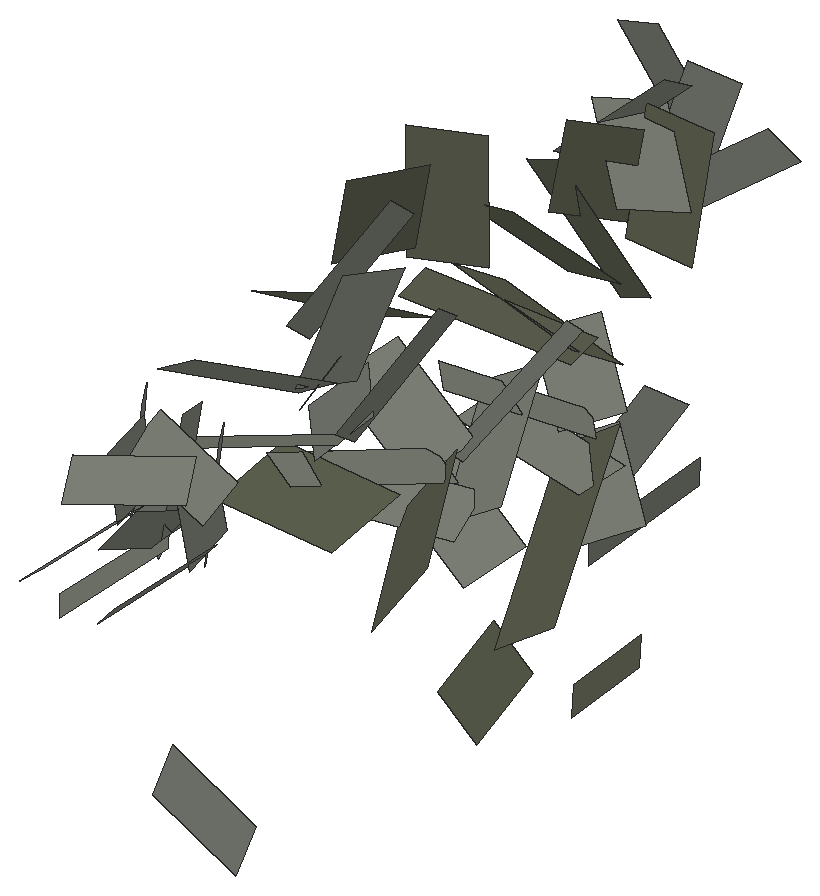
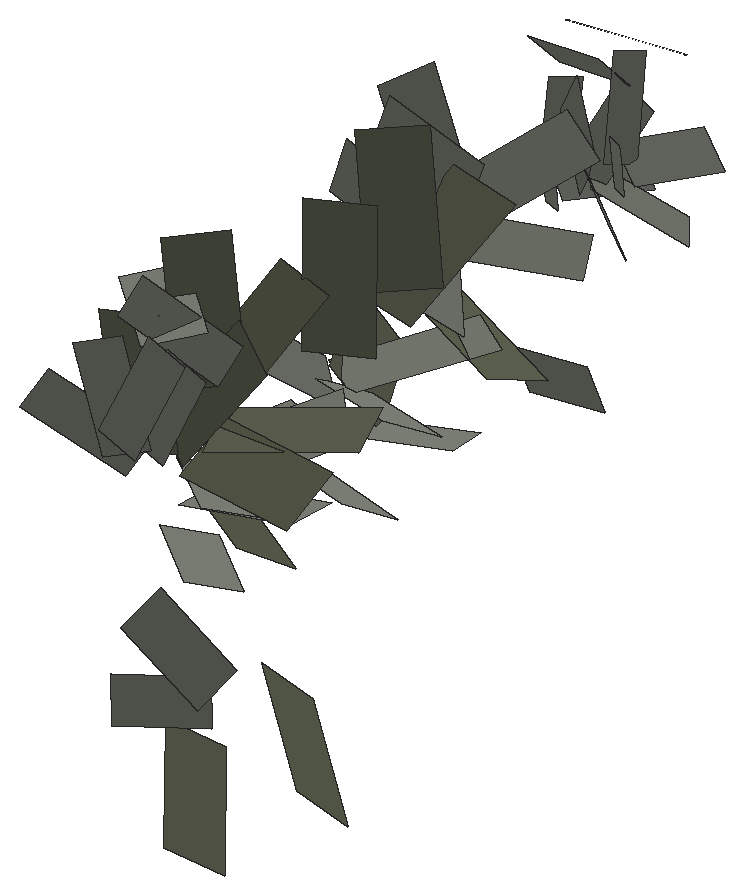
# SketchUp Ruby script. Lengths in inches.
U = 1.inch
M = Sketchup.active_model
def pt(a) = Geom::Point3d.new(a.map { |v| v * U })
def face(e, loops, mat)
  f = e.add_face(loops[0].map { |a| pt(a) })
  loops[1..].each { |l| e.add_face(l.map { |a| pt(a) }).erase! }
  f.material = f.back_material = mat if mat
  f
end
# faces: each face lists its corners as indices into pts; further lists are holes
def faces(e, pts, list, mat = nil) = list.each { |f| face(e, (f[0].is_a?(Array) ? f : [f]).map { |l| l.map { |i| pts[i] } }, mat) }
# xy, xz, yz: faces in a plane at the given z, y or x. An outline is a flat list of corners, or four numbers for a rectangle; further outlines are holes
def ring(l) = l.size == 4 ? [[l[0], l[1]], [l[2], l[1]], [l[2], l[3]], [l[0], l[3]]] : l.each_slice(2).to_a
def flat(e, list, mat, &to3) = list.each { |f| face(e, (f[0].is_a?(Array) ? f : [f]).map { |l| ring(l).map { |u, v| to3.(u, v) } }, mat) }
def xy(e, z, list, mat = nil) = flat(e, list, mat) { |x, y| [x, y, z] }
def xz(e, y, list, mat = nil) = flat(e, list, mat) { |x, z| [x, y, z] }
def yz(e, x, list, mat = nil) = flat(e, list, mat) { |y, z| [x, y, z] }
def lines(e, pts, list) = list.each { |a, b| e.add_line(pt(pts[a]), pt(pts[b])) }
# prism: a flat outline (further loops are holes) pulled along v
def prism(e, loops, v, mat = nil)
  f = face(e, loops, mat); d = Geom::Vector3d.new(v.map { |x| x * U })
  f.pushpull(f.normal.samedirection?(d) ? d.length : -d.length)
end
def box(e, o, s, mat = nil) = prism(e, [[o, [o[0] + s[0], o[1], o[2]], [o[0] + s[0], o[1] + s[1], o[2]], [o[0], o[1] + s[1], o[2]]]], [0, 0, s[2]], mat)
def at(x, y, z, deg = 0) = Geom::Transformation.translation(pt([x, y, z])) * Geom::Transformation.rotation(ORIGIN, Z_AXIS, deg.degrees)
def axes(o, x, y, z) = Geom::Transformation.new([*x, 0, *y, 0, *z, 0, *pt(o).to_a, 1])
def part(name) = M.definitions.add(name)
# library, detail: a bought-in or finely detailed component or shape, given as its bounding box
def library(name, o, s) = part(name).tap { |d| box(d.entities, o, s) }
def detail(e, o, s) = box(e.add_group.entities, o, s)
def put(e, d, t, mat = nil) = e.add_instance(d, t).tap { |i| i.material = mat if mat }
def group(e, t, mat = nil) = e.add_group.tap { |g| g.transformation = t; g.material = mat if mat }.entities
root = M.entities
M.materials.add("viburnumblaasdfas0df1w06d").color = [98, 102, 84]
M.materials.add("viburnumbladsadfasdfad0w122").color = [125, 129, 119]
c1 = part("Component\#314")
p = [[0.14,0,0],[2.58,0.05,0.25],[2.44,5.11,2.64],[0,5.05,2.39]]
faces(c1.entities,p,[[0,1,2,3]],"viburnumblaasdfas0df1w06d")
c2 = part("viburnumblad1\#2")
put(c2.entities,c1,axes([-37.25,6.23,19.31],[75.98784,0,0],[0,65.50676,0],[0,0,75.98784]))
c3 = part("Component\#315")
p = [[0.25,0,0],[2.05,0.01,0.35],[1.81,4.2,1.66],[0,4.19,1.3125]]
faces(c3.entities,p,[[0,1,2,3]],"viburnumbladsadfasdfad0w122")
c4 = part("viburnumblad2")
put(c4.entities,c3,axes([-19.23,-4.49,-32.18],[83.35428,0,0],[0,79.38502,0],[0,0,83.35428]))
put(root,c2,axes([2194.68,269.67,26.76],[-0.01129,-0.00613,-0.00067],[0.00417,-0.00777,0.01127],[-0.0047,0.00912,0.00614]))
put(root,c4,axes([2194.36,254.17,25.81],[0.0062,-0.00344,0.00762],[-0.00192,0.00879,0.00527],[-0.00787,-0.00449,0.00364]))
put(root,c4,axes([2195.61,279.33,28.08],[-0.00984,-0.00064,-0.00419],[-0.00322,-0.006,0.00808],[-0.00275,0.0086,0.00434]))
put(root,c2,axes([2197.04,271.39,24.12],[0.00188,0.00994,-0.00772],[-0.0143,-0.00023,-0.00375],[-0.00243,0.00751,0.00854]))
put(root,c2,axes([2193.96,267.38,28.05],[-0.00729,-0.01049,-0.00199],[0.00959,-0.00792,0.00787],[-0.00649,0.00328,0.00895]))
put(root,c2,axes([2197.38,270.9375,24.14],[-0.00372,0.0118,-0.00306],[-0.01362,-0.00502,-0.00283],[-0.00309,0.00191,0.01102]))
put(root,c2,axes([2196.67,267.9,13.27],[0.00499,0.00892,0.00903],[-0.00667,0.01209,-0.00778],[-0.01141,-0.0013,0.00685]))
put(root,c2,axes([2195.66,266.375,26.96],[-0.01203,-0.00093,-0.00471],[0.00029,-0.01476,0.00205],[-0.00435,0.00215,0.01023]))
put(root,c4,axes([2196.07,264.76,23.18],[0.00718,0.01175,0.00394],[-0.01195,0.00776,-0.0014],[-0.003,-0.00258,0.01303]))
put(root,c4,axes([2195.62,253.83,25.125],[0.00371,0.00412,0.00878],[-0.006,0.0085,-0.00147],[-0.00737,-0.00446,0.00446]))
put(root,c4,axes([2195.48,253.28,27.01],[-0.0062,0.00344,-0.00762],[-0.00004,-0.00961,-0.00424],[-0.0081,-0.00223,0.0048]))
put(root,c4,axes([2196.2,277.29,26.83],[-0.01027,-0.00067,-0.00437],[-0.0029,-0.0054,0.00727],[-0.00275,0.0086,0.00434]))
put(root,c4,axes([2197.32,259.9,26.98],[-0.00427,0.01006,-0.00619],[-0.01054,-0.00775,-0.00533],[-0.00749,0.00313,0.01026]))
put(root,c4,axes([2196.43,253.22,26],[-0.00506,0.00898,-0.002],[-0.00471,-0.00455,-0.00828],[-0.00753,-0.00286,0.00529]))
put(root,c4,axes([2196.67,260.61,28.44],[-0.00935,0.0021,-0.00891],[-0.00409,-0.01235,0.00138],[-0.00819,0.00377,0.00948]))
put(root,c4,axes([2197.66,264.6875,21.89],[-0.00305,0.01398,0.00068],[-0.01364,-0.00282,-0.0033],[-0.00279,-0.00128,0.01326]))
put(root,c4,axes([2194.46,275.59,16.81],[-0.00173,-0.0098,0.00563],[0.00735,0.00343,0.00822],[-0.00865,0.00481,0.00572]))
put(root,c4,axes([2194.93,254.49,26.95],[0.00095,-0.00927,-0.00479],[0.00517,-0.00382,0.00808],[-0.00874,-0.00294,0.00329]))
put(root,c4,axes([2194.1,275.0625,28.37],[0.00162,-0.00936,0.00394],[0.00963,0.00389,0.00496],[-0.00566,0.00263,0.0077]))
put(root,c2,axes([2197.62,273.6,25.08],[-0.00938,0.00386,-0.00599],[-0.00819,-0.00718,0.008],[-0.00057,0.00892,0.00623]))
put(root,c2,axes([2198.51,259.2,23.77],[0.00387,0.01311,0.00437],[-0.0121,0.00667,-0.00928],[-0.00906,-0.00102,0.01108]))
put(root,c4,axes([2197.77,264.79,23.78],[-0.01149,0.00801,-0.00297],[-0.00766,-0.01186,-0.00235],[-0.00352,-0.00017,0.01315]))
put(root,c4,axes([2196.13,260.3125,25.88],[0.00916,0.00784,0.00642],[-0.00492,0.00961,-0.00471],[-0.00802,0.00094,0.01029]))
put(root,c4,axes([2195.07,261.02,26.84],[0.00935,-0.0021,0.00891],[0.00182,0.01184,0.00088],[-0.00893,0.00067,0.00953]))
put(root,c4,axes([2194.54,262.14,28.43],[0.00445,-0.01048,0.00645],[0.00766,0.00772,0.00727],[-0.00963,0.0013,0.00876]))
put(root,c4,axes([2194.7,274.57,15.69],[0.00508,-0.00494,0.00777],[0.00608,0.00946,0.00204],[-0.00795,0.00351,0.00743]))
put(root,c2,axes([2197.29,272.64,25.9],[-0.0112,0.0013,-0.00343],[-0.00292,-0.0124,0.00476],[-0.00244,0.00473,0.0094]))
put(root,c4,axes([2197.59,265.23,20.14],[0.00689,0.01128,0.00378],[-0.0129,0.00838,-0.00151],[-0.003,-0.00258,0.01303]))
put(root,c4,axes([2195.87,278.78,26.76],[-0.00898,-0.00541,0.00233],[0.00475,-0.00369,0.00928],[-0.0037,0.00829,0.00425]))
put(root,c2,axes([2197.33,271.28,12.77],[0.00721,0.00805,0.00636],[-0.00379,0.01064,-0.00917],[-0.00973,0.00288,0.00737]))
put(root,c4,axes([2196.94,270.48,22.66],[0.00933,0.00906,0.00093],[-0.00886,0.00934,-0.00204],[-0.00208,0.00083,0.01284]))
put(root,c4,axes([2195.59,254.85,25.73],[0.00506,-0.00898,0.002],[0.00284,0.00386,0.00969],[-0.00844,-0.00386,0.00315]))
put(root,c4,axes([2198.22,269.8,21.37],[0.00055,0.01289,-0.00188],[-0.01292,0.00032,-0.00165],[-0.00158,0.00193,0.01279]))
put(root,c4,axes([2196.53,254.74,24.8],[0.00595,-0.0033,0.00732],[-0.00208,0.00949,0.0057],[-0.00787,-0.00449,0.00364]))
put(root,c4,axes([2198.5,270.2,23.1],[-0.00854,0.00917,-0.00359],[-0.00964,-0.00875,0.0006],[-0.00199,0.00305,0.01252]))
put(root,c2,axes([2196.11,274.12,26.82],[-0.00897,-0.00759,0.00065],[0.00732,-0.00776,0.00825],[-0.00418,0.00599,0.00812]))
put(root,c4,axes([2196.32,254.53,26.66],[-0.00371,-0.00412,-0.00878],[0.00371,-0.00856,0.0023],[-0.0086,-0.00227,0.00398]))
put(root,c4,axes([2196.44,265.71,21.5625],[0.0132,0.00264,0.00489],[-0.00375,0.01436,0.00234],[-0.00402,-0.00331,0.01259]))
put(root,c2,axes([2197.16,275.68,25.13],[-0.01138,-0.00264,0.00129],[0.00289,-0.0057,0.01174],[-0.00153,0.01008,0.00426]))
put(root,c4,axes([2197.46,254.11,26.08],[-0.00487,0.00336,-0.00745],[-0.00004,-0.00961,-0.00424],[-0.00872,-0.00185,0.00395]))
put(root,c4,axes([2195.68,277.9,25.74],[-0.00274,-0.00672,0.00719],[0.01014,0.00172,0.00518],[-0.00429,0.00766,0.00474]))
put(root,c4,axes([2198.91,251.03,29.23],[-0.00345,0.00905,0.004],[-0.00954,-0.00184,-0.00399],[-0.00252,-0.00485,0.0079]))
put(root,c4,axes([2196.28,262.09,27.74],[-0.00306,-0.01272,0.00021],[0.00831,-0.00183,0.01011],[-0.0097,0.00247,0.00842]))
put(root,c4,axes([2198.12,269.98,19.63],[0.00895,0.00869,0.00089],[-0.00957,0.01008,-0.0022],[-0.00208,0.00083,0.01284]))
put(root,c4,axes([2198.4,271.56,29.91],[0.00912,0.00933,-0.00467],[-0.01186,0.01016,-0.00285],[0.00181,0.00573,0.01291]))
put(root,c4,axes([2198.84,251.88,28.19],[0.00404,0.00727,0.00631],[-0.0093,0.00487,0.00025],[-0.00255,-0.00567,0.00738]))
put(root,c4,axes([2197.03,255.15,25.95],[0.00099,-0.00968,-0.005],[0.00466,-0.00344,0.00728],[-0.00874,-0.00294,0.00329]))
put(root,c4,axes([2195.97,266.56,23.375],[0.01149,-0.00801,0.00297],[0.00658,0.01147,0.00547],[-0.00527,-0.00304,0.01219]))
put(root,c4,axes([2196.52,261.66,26.05],[0.00502,-0.00971,0.00503],[0.00766,0.00772,0.00727],[-0.00909,0.00016,0.0094]))
put(root,c4,axes([2199.24,252.69,16.625],[0.00409,0.00375,0.00971],[-0.00938,0.00585,0.00169],[-0.00452,-0.00876,0.00528]))
put(root,c2,axes([2198.06,266.86,16.89],[0.01357,-0.0015,0.0077],[-0.00069,0.01762,0.00453],[-0.00774,-0.0037,0.01228]))
put(root,c2,axes([2199.37,259.74,21.3],[0.00862,0.00382,0.01082],[-0.00301,0.01604,-0.00327],[-0.01117,-0.00026,0.009]))
